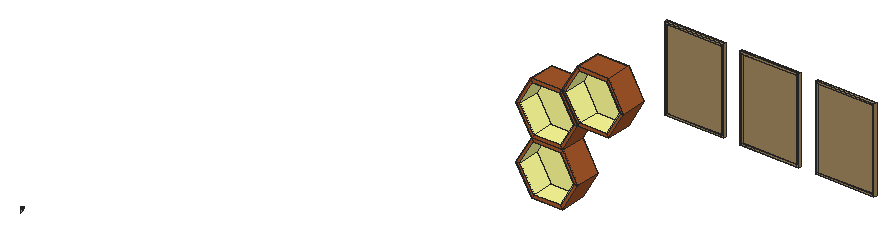
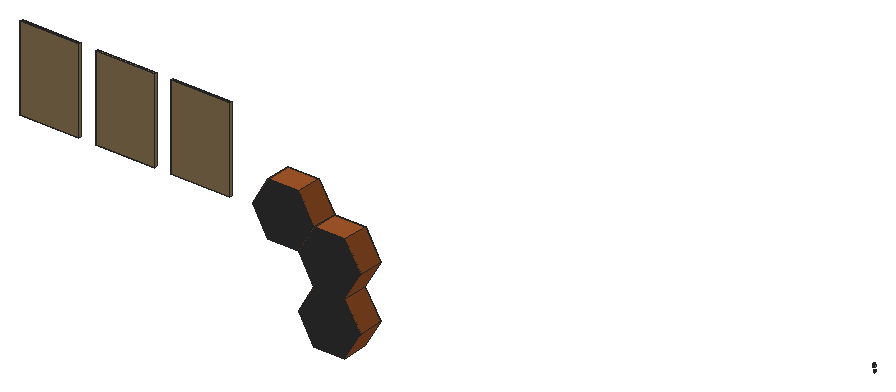
# SketchUp Ruby script. Lengths in inches.
U = 1.inch
M = Sketchup.active_model
def pt(a) = Geom::Point3d.new(a.map { |v| v * U })
def face(e, loops, mat)
  f = e.add_face(loops[0].map { |a| pt(a) })
  loops[1..].each { |l| e.add_face(l.map { |a| pt(a) }).erase! }
  f.material = f.back_material = mat if mat
  f
end
# faces: each face lists its corners as indices into pts; further lists are holes
def faces(e, pts, list, mat = nil) = list.each { |f| face(e, (f[0].is_a?(Array) ? f : [f]).map { |l| l.map { |i| pts[i] } }, mat) }
# xy, xz, yz: faces in a plane at the given z, y or x. An outline is a flat list of corners, or four numbers for a rectangle; further outlines are holes
def ring(l) = l.size == 4 ? [[l[0], l[1]], [l[2], l[1]], [l[2], l[3]], [l[0], l[3]]] : l.each_slice(2).to_a
def flat(e, list, mat, &to3) = list.each { |f| face(e, (f[0].is_a?(Array) ? f : [f]).map { |l| ring(l).map { |u, v| to3.(u, v) } }, mat) }
def xy(e, z, list, mat = nil) = flat(e, list, mat) { |x, y| [x, y, z] }
def xz(e, y, list, mat = nil) = flat(e, list, mat) { |x, z| [x, y, z] }
def yz(e, x, list, mat = nil) = flat(e, list, mat) { |y, z| [x, y, z] }
def lines(e, pts, list) = list.each { |a, b| e.add_line(pt(pts[a]), pt(pts[b])) }
# prism: a flat outline (further loops are holes) pulled along v
def prism(e, loops, v, mat = nil)
  f = face(e, loops, mat); d = Geom::Vector3d.new(v.map { |x| x * U })
  f.pushpull(f.normal.samedirection?(d) ? d.length : -d.length)
end
def box(e, o, s, mat = nil) = prism(e, [[o, [o[0] + s[0], o[1], o[2]], [o[0] + s[0], o[1] + s[1], o[2]], [o[0], o[1] + s[1], o[2]]]], [0, 0, s[2]], mat)
def at(x, y, z, deg = 0) = Geom::Transformation.translation(pt([x, y, z])) * Geom::Transformation.rotation(ORIGIN, Z_AXIS, deg.degrees)
def axes(o, x, y, z) = Geom::Transformation.new([*x, 0, *y, 0, *z, 0, *pt(o).to_a, 1])
def part(name) = M.definitions.add(name)
# library, detail: a bought-in or finely detailed component or shape, given as its bounding box
def library(name, o, s) = part(name).tap { |d| box(d.entities, o, s) }
def detail(e, o, s) = box(e.add_group.entities, o, s)
def put(e, d, t, mat = nil) = e.add_instance(d, t).tap { |i| i.material = mat if mat }
def group(e, t, mat = nil) = e.add_group.tap { |g| g.transformation = t; g.material = mat if mat }.entities
root = M.entities
M.materials.add("509740_G").color = [165, 87, 41]
M.materials.add("Laura_Hair").color = [160, 135, 94]
M.materials.add("[Color_007]").color = [58, 58, 58]
M.materials.add("[Color_E04]").color = [255, 255, 153]
M.materials.add("green").color = [174, 139, 102]
M.materials.add("vio").color = [206, 114, 100]
c1 = library("3DGeom~100_Defintion",[-500,-440.78,-130.77],[1000,881.57,261.54])
c2 = part("3DGeom~101_Defintion")
p = [[450.26,-438.5,-76.98],[473.93,-418.23,-130.77],[473.01,-420.54,-57.59],[450.72,-437.34,-113.57],[473.93,-418.23,-130.77],[450.26,-438.5,-76.98],
  [473.93,-418.23,-130.77],[450.72,-437.34,-113.57],[460.6,-429.08,-126.5],[473.01,-420.54,-57.59],[473.93,-418.23,-130.77],[496.21,-401.44,-74.78],
  [473.93,-418.23,-130.77],[487.14,-407.6875,-125.23],[496.68,-400.28,-111.37],[473.93,-418.23,-130.77],[496.68,-400.28,-111.37],[450.72,-437.34,-113.57],
  [450.26,-438.5,-76.98],[446.9375,-440.78,-95.45],[496.68,-400.28,-111.37],[500,-397.99,-92.9],[450.26,-438.5,-76.98],[473.01,-420.54,-57.59],
  [459.8,-431.09,-63.125],[473.01,-420.54,-57.59],[486.33,-409.69,-61.85],[-483.04,428.3125,67.76],[-497.53,394.8,97.99],[-487.96,391.61,113.91],
  [-483.04,428.3125,67.76],[-487.96,391.61,113.91],[-473.84,395.01,125.91],[-483.04,428.3125,67.76],[-500,403.73,82.41],[-497.53,394.8,97.99],
  [-483.04,428.3125,67.76],[-473.84,395.01,125.91],[-458.96,404.09,130.77],[-483.04,428.3125,67.76],[-494.7,415.99,71.34],[-483.04,428.3125,67.76],
  [-458.96,404.09,130.77],[-447.31,416.41,127.18],[-483.04,428.3125,67.76],[-447.31,416.41,127.18],[-442,428.67,116.12],[-483.04,428.3125,67.76],
  [-444.47,437.6,100.54],[-454.05,440.79,84.62],[-483.04,428.3125,67.76],[-454.05,440.79,84.62],[-468.16,437.39,72.62],[-483.04,428.3125,67.76],
  [-442,428.67,116.12],[-444.47,437.6,100.54]]
faces(c2.entities,p,[[0,1,2],[3,4,5],[6,7,8],[9,10,11],[12,13,14],[11,15,16],[17,18,19],[11,20,21],
  [22,23,24],[25,11,26],[27,28,29],[30,31,32],[33,34,35],[36,37,38],[39,40,34],[41,42,43],
  [44,45,46],[47,48,49],[50,51,52],[53,54,55]],"green")
c3 = part("3DGeom~221_Defintion")
p = [[192.89,-154.12,-424.75],[-160.54,-146.25,-441.73],[24.02,0,-500],[348.39,12.78,-359.13],[-312.36,-12.78,-390.87],[-151.29,154.12,-441.28],
  [202.15,146.25,-424.3],[348.39,12.78,-359.13],[-14.3,-279.72,-376.55],[-302.09,-253.31,-265.09],[-389.74,-176.26,-235.73],[-389.74,-176.26,-235.73],
  [-429.08,84.92,-237.62],[-429.08,84.92,-237.62],[-286.06,266.94,-264.32],[50.33,279.72,-373.45],[50.33,279.72,-373.45],[-286.06,266.94,-264.32],
  [310.08,-266.94,-235.68],[449.88,-84.92,-195.39],[310.08,-266.94,-235.68],[192.89,-154.12,-424.75],[192.89,-154.12,-424.75],[348.39,12.78,-359.13],
  [410.54,176.26,-197.28],[202.15,146.25,-424.3],[326.11,253.31,-234.91],[50.33,279.72,-373.45],[202.15,146.25,-424.3],[326.11,253.31,-234.91],
  [-312.36,-12.78,-390.87],[-389.74,-176.26,-235.73],[-457.125,-119.85,-147.25],[-312.36,-12.78,-390.87],[-429.08,84.92,-237.62],[87.19,-377.43,-212.82],
  [-217.65,-330.375,-227.46],[-14.3,-279.72,-376.55],[310.08,-266.94,-235.68],[87.19,-377.43,-212.82],[-217.65,-330.375,-227.46],[326.11,253.31,-234.91],
  [50.33,279.72,-373.45],[238.45,330.375,-205.55],[50.33,279.72,-373.45],[-286.06,266.94,-264.32],[-66.39,377.43,-220.19],[238.45,330.375,-205.55],
  [50.33,279.72,-373.45],[-66.39,377.43,-220.19],[469.14,119.85,-102.75],[-302.09,-253.31,-265.09],[-217.65,-330.375,-227.46],[-362.6875,-292.5,-17.42],
  [-302.09,-253.31,-265.09],[-362.6875,-292.5,-17.42],[-286.06,266.94,-264.32],[-479.41,120.6875,-23.03],[-286.06,266.94,-264.32],[-344.18,308.23,-16.53],
  [-286.06,266.94,-264.32],[-344.18,308.23,-16.53],[-486.1875,-99.2,-23.36],[344.18,-308.23,16.53],[87.19,-377.43,-212.82],[310.08,-266.94,-235.68],
  [479.41,-120.6875,23.03],[344.18,-308.23,16.53],[-362.6875,-292.5,-17.42],[362.6875,292.5,17.42],[238.45,330.375,-205.55],[-217.65,-330.375,-227.46],
  [-159.06,-386.79,-132.93],[-362.6875,-292.5,-17.42],[87.19,-377.43,-212.82],[-217.65,-330.375,-227.46],[-116.72,413.19,-5.61],[171.07,386.79,-117.07],
  [116.72,-413.19,5.61],[87.19,-377.43,-212.82],[344.18,-308.23,16.53],[87.19,-377.43,-212.82],[362.6875,292.5,17.42],[486.1875,99.2,23.36],
  [-362.6875,-292.5,-17.42],[-142.01,-407.43,-6.82],[142.01,407.43,6.82],[362.6875,292.5,17.42],[-469.14,-119.85,102.75],[-362.6875,-292.5,-17.42],
  [-449.88,84.92,195.39],[-344.18,308.23,-16.53],[-171.07,-386.79,117.07],[-238.45,-330.375,205.55],[-238.45,-330.375,205.55],[-326.11,-253.31,234.91],
  [-362.6875,-292.5,-17.42],[-410.54,-176.26,197.28],[-362.6875,-292.5,-17.42],[-326.11,-253.31,234.91],[-362.6875,-292.5,-17.42],[-344.18,308.23,-16.53],
  [-310.08,266.94,235.68],[-310.08,266.94,235.68],[66.39,-377.43,220.2],[-310.08,266.94,235.68],[-87.19,377.43,212.82],[286.06,-266.94,264.32],
  [286.06,-266.94,264.32],[344.18,-308.23,16.53],[159.06,386.79,132.93],[362.6875,292.5,17.42],[429.08,-84.92,237.62],[286.06,-266.94,264.32],
  [457.125,119.85,147.25],[389.74,176.26,235.73],[302.09,253.31,265.09],[217.65,330.375,227.46],[217.65,330.375,227.46],[362.6875,292.5,17.42],
  [-50.33,-279.72,373.45],[-50.33,-279.72,373.45],[14.3,279.72,376.55],[14.3,279.72,376.55],[217.65,330.375,227.46],[-348.39,-12.78,359.13],
  [-310.08,266.94,235.68],[-348.39,-12.78,359.13],[-348.39,-12.78,359.13],[-326.11,-253.31,234.91],[-202.15,-146.25,424.3],[-326.11,-253.31,234.91],
  [-238.45,-330.375,205.55],[-238.45,-330.375,205.55],[-50.33,-279.72,373.45],[-87.19,377.43,212.82],[-310.08,266.94,235.68],[-192.89,154.12,424.75],
  [-87.19,377.43,212.82],[14.3,279.72,376.55],[151.29,-154.12,441.28],[66.39,-377.43,220.2],[66.39,-377.43,220.2],[286.06,-266.94,264.32],
  [217.65,330.375,227.46],[160.54,146.25,441.73],[217.65,330.375,227.46],[302.09,253.31,265.09],[-348.39,-12.78,359.13],[-326.11,-253.31,234.91],
  [-202.15,-146.25,424.3],[312.36,12.78,390.87],[-310.08,266.94,235.68],[-348.39,-12.78,359.13],[-192.89,154.12,424.75],[302.09,253.31,265.09],
  [312.36,12.78,390.87],[389.74,176.26,235.73],[312.36,12.78,390.87],[286.06,-266.94,264.32],[429.08,-84.92,237.62],[312.36,12.78,390.87],
  [286.06,-266.94,264.32],[302.09,253.31,265.09],[312.36,12.78,390.87],[-348.39,-12.78,359.13],[-24.02,0,500],[312.36,12.78,390.87]]
faces(c3.entities,p,[[0,1,2],[3,0,2],[2,1,4],[2,4,5],[6,2,5],[7,2,6],[8,9,1],[0,8,1],
  [1,9,10],[1,11,4],[5,4,12],[5,13,14],[6,5,15],[16,5,17],[18,8,0],[19,20,21],
  [19,22,23],[24,23,25],[26,6,27],[24,28,29],[30,31,32],[33,32,34],[35,36,37],[38,39,8],
  [8,40,9],[41,42,43],[44,45,46],[47,48,49],[50,19,23],[50,23,24],[51,52,53],[31,54,55],
  [56,34,57],[58,57,59],[49,60,61],[34,32,62],[34,62,57],[63,64,65],[66,67,20],[32,31,68],
  [66,20,19],[24,29,69],[29,70,69],[71,72,73],[74,72,75],[49,61,76],[47,49,77],[77,49,76],
  [78,72,79],[80,78,81],[47,77,82],[50,24,69],[83,66,19],[83,19,50],[62,32,84],[78,85,72],
  [72,85,73],[77,86,87],[77,76,86],[83,50,69],[88,62,89],[57,62,88],[57,88,90],[91,57,90],
  [85,92,73],[92,93,73],[94,95,96],[97,88,98],[99,97,100],[101,90,102],[76,61,103],[104,85,78],
  [104,92,85],[76,105,106],[86,76,106],[107,104,78],[108,78,109],[86,110,111],[86,106,110],[112,113,67],
  [112,67,66],[114,83,69],[115,114,69],[116,115,69],[117,116,69],[110,118,119],[114,112,66],[114,66,83],
  [90,88,97],[120,93,92],[121,92,104],[110,106,122],[110,123,124],[115,112,114],[90,97,125],[126,90,127],
  [128,97,129],[130,131,132],[130,133,134],[135,136,137],[138,137,139],[140,134,141],[140,142,143],[144,139,145],
  [146,145,147],[148,149,150],[115,151,112],[152,153,154],[155,156,157],[158,159,160],[161,140,162],[163,145,164],
  [137,165,130],[166,130,134],[166,134,140],[139,137,166],[139,166,145],[145,140,167],[137,130,166],[145,166,140]],"vio")
c4 = library("3DGeom~121_Defintion",[-425.32,-500,-417.04],[850.64,1000,834.08])
c5 = part("3DGeom~122_Defintion")
p = [[-352.95,-477.04,-406.33],[-422.05,-474.42,-360.32],[-383.91,-455.37,-417.04],[-352.95,-477.04,-406.33],[-383.91,-455.37,-417.04],[-365.48,-464.73,-416.07],
  [-383.91,-455.37,-417.04],[-422.05,-474.42,-360.32],[-418.46,-454.05,-394.04],[-383.91,-455.37,-417.04],[-418.46,-454.05,-394.04],[-403.3,-451.46,-408.98],
  [-356.54,-497.41,-372.61],[-422.05,-474.42,-360.32],[-352.95,-477.04,-406.33],[-356.54,-497.41,-372.61],[-352.95,-477.04,-406.33],[-349.67,-489,-390.42],
  [-422.05,-474.42,-360.32],[-425.32,-462.46,-376.23],[-418.46,-454.05,-394.04],[-391.09,-496.09,-349.6],[-356.54,-497.41,-372.61],[-371.7,-500,-357.67],
  [-391.09,-496.09,-349.6],[-422.05,-474.42,-360.32],[-356.54,-497.41,-372.61],[-422.05,-474.42,-360.32],[-391.09,-496.09,-349.6],[-409.52,-486.73,-350.57],
  [376.78,485.85,408.43],[420.34,458.37,345.52],[409.52,472.35,336.91],[376.78,485.85,408.43],[409.52,472.35,336.91],[395.77,486.26,339.03],
  [376.78,485.85,408.43],[395.77,486.26,339.03],[382.76,496.38,351.32],[376.78,485.85,408.43],[425.32,448.07,362.5625],[420.34,458.37,345.52],
  [376.78,485.85,408.43],[382.76,496.38,351.32],[373.99,500,370.48],[376.78,485.85,408.43],[423.13,444.22,383.47],[376.78,485.85,408.43],
  [373.99,500,370.48],[371.8,496.14,391.39],[376.78,485.85,408.43],[414.36,447.84,402.63],[423.13,444.22,383.47],[376.78,485.85,408.43],
  [401.35,457.96,414.92],[414.36,447.84,402.63],[376.78,485.85,408.43],[387.6,471.87,417.04],[401.35,457.96,414.92]]
faces(c5.entities,p,[[0,1,2],[3,4,5],[6,7,8],[9,10,11],[12,13,14],[15,16,17],[18,19,20],[21,22,23],
  [24,25,26],[27,28,29],[30,31,32],[33,34,35],[36,37,38],[39,40,41],[42,43,44],[45,46,40],
  [47,48,49],[50,51,52],[53,54,55],[56,57,58]],"green")
c6 = part("3DGeom~227_Defintion")
p = [[-46.82,-86.11,-495.11],[-183.22,-312.53,-297.48],[-255.21,-122.37,-414.37],[57.41,-270.66,-390.71],[148.25,12.96,-485.1875],[-138.51,121.52,-466.84],
  [-25.88,178.72,-461.11],[282.66,-156.27,-379.26],[277.73,148.29,-387.25],[48.875,256.85,-404.57],[-258.82,100.58,-420.23],[-193.08,296.58,-313.48],
  [-421.09,-86.11,-264.6],[-421.09,-86.11,-264.6],[-354.59,121.52,-333.75],[-255.21,-122.37,-414.37],[-183.22,-312.53,-297.48],[-374.76,-270.66,-124.54],
  [-255.21,-122.37,-414.37],[-421.09,-86.11,-264.6],[65.73,334.98,-312.37],[57.41,-270.66,-390.71],[-62.14,-418.95,-100.89],[-183.22,-312.53,-297.48],
  [57.41,-270.66,-390.71],[146.25,-382.69,-181.63],[146.25,-382.69,-181.63],[432.17,0,-266.17],[306.92,283.62,-227.56],[432.17,0,-266.17],
  [277.73,148.29,-387.25],[306.92,283.62,-227.56],[341.32,-283.625,-171.7],[146.25,-382.69,-181.63],[432.17,0,-266.17],[341.32,-283.625,-171.7],
  [282.66,-156.27,-379.26],[-354.59,121.52,-333.75],[-500,12.96,-85.92],[-354.59,121.52,-333.75],[-400.15,178.72,-230.6],[-400.15,178.72,-230.6],
  [-383.29,256.85,-138.4],[-193.08,296.58,-313.48],[-383.29,256.85,-138.4],[-308.54,334.98,-81.86],[-193.08,296.58,-313.48],[-195.91,392.18,-76.125],
  [-193.08,296.58,-313.48],[-75.6,413.11,-122.74],[-193.08,296.58,-313.48],[20.17,392.18,-209.21],[65.73,334.98,-312.37],[-193.08,296.58,-313.48],
  [-193.08,296.58,-313.48],[306.92,283.62,-227.56],[65.73,334.98,-312.37],[-183.22,-312.53,-297.48],[-228.01,-382.69,48.88],[-183.22,-312.53,-297.48],
  [-228.01,-382.69,48.88],[-374.76,-270.66,-124.54],[432.17,0,-266.17],[470.8,-148.29,-73.77],[341.32,-283.625,-171.7],[465.88,156.27,-81.77],
  [432.17,0,-266.17],[306.92,283.62,-227.56],[432.17,0,-266.17],[-465.88,-156.27,81.77],[-470.8,148.29,73.77],[-383.29,256.85,-138.4],
  [228.01,382.69,-48.88],[306.92,283.62,-227.56],[228.01,382.69,-48.88],[306.92,283.62,-227.56],[75.6,-413.11,122.74],[195.91,-392.18,76.125],
  [341.32,-283.625,-171.7],[341.32,-283.625,-171.7],[308.54,-334.98,81.86],[308.54,-334.98,81.86],[341.32,-283.625,-171.7],[-383.29,256.85,-138.4],
  [-341.32,283.625,171.7],[-383.29,256.85,-138.4],[-341.32,283.625,171.7],[-308.54,334.98,-81.86],[-228.01,-382.69,48.88],[-306.92,-283.62,227.56],
  [62.14,418.95,100.89],[-20.17,-392.18,209.21],[-228.01,-382.69,48.88],[-432.17,0,266.17],[-341.32,283.625,171.7],[-146.25,382.69,181.63],
  [500,-12.96,85.92],[374.76,270.66,124.54],[228.01,382.69,-48.88],[383.29,-256.85,138.4],[308.54,-334.98,81.86],[374.76,270.66,124.54],
  [-228.01,-382.69,48.88],[-65.73,-334.98,312.37],[-228.01,-382.69,48.88],[-65.73,-334.98,312.37],[-306.92,-283.62,227.56],[-282.66,156.27,379.26],
  [-282.66,156.27,379.26],[-341.32,283.625,171.7],[193.08,-296.58,313.48],[-277.73,-148.29,387.25],[-277.73,-148.29,387.25],[383.29,-256.85,138.4],
  [400.15,-178.72,230.6],[421.09,86.11,264.6],[183.22,312.53,297.48],[374.76,270.66,124.54],[183.22,312.53,297.48],[193.08,-296.58,313.48],
  [-341.32,283.625,171.7],[-282.66,156.27,379.26],[-57.41,270.66,390.71],[-341.32,283.625,171.7],[-57.41,270.66,390.71],[-146.25,382.69,181.63],
  [-57.41,270.66,390.71],[-65.73,-334.98,312.37],[-306.92,-283.62,227.56],[-65.73,-334.98,312.37],[-48.875,-256.85,404.57],[-306.92,-283.62,227.56],
  [-277.73,-148.29,387.25],[400.15,-178.72,230.6],[354.59,-121.52,333.75],[193.08,-296.58,313.48],[354.59,-121.52,333.75],[255.21,122.37,414.37],
  [354.59,-121.52,333.75],[421.09,86.11,264.6],[183.22,312.53,297.48],[255.21,122.37,414.37],[-432.17,0,266.17],[-148.25,-12.96,485.1875],
  [-432.17,0,266.17],[-57.41,270.66,390.71],[255.21,122.37,414.37],[183.22,312.53,297.48],[193.08,-296.58,313.48],[25.88,-178.72,461.11],
  [193.08,-296.58,313.48],[138.51,-121.52,466.84],[193.08,-296.58,313.48],[258.82,-100.58,420.23],[193.08,-296.58,313.48],[354.59,-121.52,333.75],
  [193.08,-296.58,313.48],[255.21,122.37,414.37],[354.59,-121.52,333.75],[46.82,86.11,495.11],[-57.41,270.66,390.71],[-57.41,270.66,390.71],
  [255.21,122.37,414.37],[255.21,122.37,414.37]]
faces(c6.entities,p,[[0,1,2],[0,3,1],[4,3,0],[5,0,2],[6,0,5],[6,4,0],[4,7,3],[8,7,4],
  [9,4,6],[9,8,4],[5,2,10],[5,10,11],[6,5,11],[9,6,11],[10,2,12],[10,13,14],
  [10,14,11],[15,16,17],[18,17,19],[20,8,9],[20,9,11],[21,22,23],[24,25,22],[7,26,3],
  [8,27,7],[28,29,30],[20,31,8],[7,32,33],[34,35,36],[37,19,38],[39,38,40],[14,41,11],
  [40,42,43],[44,45,46],[45,47,48],[47,49,50],[51,52,53],[49,51,54],[51,55,56],[57,22,58],
  [59,60,61],[62,63,64],[65,63,66],[67,65,68],[19,17,69],[19,69,38],[40,38,70],[40,70,71],
  [72,65,73],[51,74,75],[49,74,51],[25,76,22],[25,77,76],[78,77,25],[79,80,77],[63,81,82],
  [83,70,84],[85,86,87],[17,88,89],[17,89,69],[49,90,74],[47,90,49],[22,91,92],[22,76,91],
  [38,69,93],[38,93,70],[45,94,95],[45,95,47],[65,96,63],[97,96,65],[98,97,65],[47,95,90],
  [63,99,100],[96,99,63],[90,101,74],[102,91,103],[104,105,106],[70,93,107],[70,108,109],[76,77,110],
  [77,80,110],[69,89,111],[69,112,93],[80,113,110],[96,114,99],[115,114,96],[97,115,96],[90,116,117],
  [95,116,90],[91,76,110],[118,115,97],[99,114,119],[120,121,122],[123,124,125],[95,126,116],[127,91,110],
  [128,129,130],[131,130,132],[133,134,135],[115,136,114],[137,138,139],[140,141,115],[142,132,143],[144,143,121],
  [145,146,147],[130,129,148],[149,130,150],[151,149,152],[153,151,154],[155,153,156],[157,153,158],[121,143,159],
  [121,159,160],[132,130,149],[132,149,143],[161,159,162],[159,153,163],[159,151,153],[143,149,151],[143,151,159]],"vio")
c7 = part("Group\#32")
xy(c7.entities,0,[[3.62,0,10.87,5.91]],"509740_G")
xy(c7.entities,0.79,[[4.08,0,10.41,5.12]],"[Color_E04]")
xy(c7.entities,11.8125,[[4.08,0,10.41,5.12]],"[Color_E04]")
xy(c7.entities,12.6,[[3.62,0,10.87,5.91]],"509740_G")
xz(c7.entities,0,[[3.62,0,4.08,0.79,0.91,6.3,0,6.3],[3.62,0,10.87,0,10.41,0.79,4.08,0.79],[10.87,0,14.49,6.3,13.58,6.3,10.41,0.79],[0,6.3,0.91,6.3,4.08,11.8125,3.62,12.6],[13.58,6.3,14.49,6.3,10.87,12.6,10.41,11.8125],
  [4.08,11.8125,10.41,11.8125,10.87,12.6,3.62,12.6]],"509740_G")
xz(c7.entities,5.12,[[4.08,0.79,10.41,0.79,13.58,6.3,10.41,11.8125,4.08,11.8125,0.91,6.3]],"[Color_E04]")
xz(c7.entities,5.91,[[3.62,0,0,6.3,3.62,12.6,10.87,12.6,14.49,6.3,10.87,0]],"[Color_007]")
p = [[0,5.91,6.3],[3.62,5.91,0],[3.62,0,0],[0,0,6.3],[10.87,5.91,0],[14.49,5.91,6.3],
  [14.49,0,6.3],[10.87,0,0],[0.91,0,6.3],[4.08,0,0.79],[4.08,5.12,0.79],[0.91,5.12,6.3],
  [10.41,0,0.79],[13.58,0,6.3],[13.58,5.12,6.3],[10.41,5.12,0.79],[3.62,5.91,12.6],[3.62,0,12.6],
  [4.08,0,11.8125],[4.08,5.12,11.8125],[10.41,0,11.8125],[10.41,5.12,11.8125],[10.87,5.91,12.6],[10.87,0,12.6]]
faces(c7.entities,p,[[0,1,2,3],[4,5,6,7],[16,0,3,17],[5,22,23,6]],"509740_G")
faces(c7.entities,p,[[8,9,10,11],[12,13,14,15],[18,8,11,19],[13,20,21,14]],"[Color_E04]")
c8 = part("WALL SHELVES 01")
g1 = group(c8.entities,at(13.71,-9.84,19.85))
put(g1,c7,at(0,0,0))
put(g1,c7,at(10.87,0,6.3))
put(g1,c7,at(21.73,0,0))
c9 = part("Plant Wall Art")
g2 = group(c9.entities,at(1.72,0.59,0))
xy(g2,0,[[0,-0.59,13.78,0]],"Laura_Hair")
xy(g2,0.39,[[0.39,-0.59,13.39,-0.39]],"Laura_Hair")
xy(g2,19.29,[[0.39,-0.59,13.39,-0.39]],"Laura_Hair")
xy(g2,19.69,[[0,-0.59,13.78,0]],"Laura_Hair")
xz(g2,-0.59,[[[0,0,13.78,19.69],[0.39,0.39,13.39,19.29]]],"Laura_Hair")
xz(g2,0,[[0,0,13.78,19.69]],"Laura_Hair")
yz(g2,0,[[-0.59,0,0,19.69]],"Laura_Hair")
yz(g2,0.39,[[-0.59,0.39,-0.39,19.29]],"Laura_Hair")
yz(g2,13.39,[[-0.59,0.39,-0.39,19.29]],"Laura_Hair")
yz(g2,13.78,[[-0.59,0,0,19.69]],"Laura_Hair")
p = [[13.39,0,0.39],[13.39,-0.39,0.39],[13.39,0,19.29],[13.39,-0.39,19.29],[0.39,0,0.39],[0.39,-0.39,0.39],
  [0.39,0,19.29],[0.39,-0.39,19.29]]
lines(g2,p,[[0,1],[2,3],[4,5],[6,7]])
g3 = group(c9.entities,at(19.43,0.59,0))
xy(g3,0,[[0,-0.59,13.78,0]],"Laura_Hair")
xy(g3,0.39,[[0.39,-0.59,13.39,-0.39]],"Laura_Hair")
xy(g3,19.29,[[0.39,-0.59,13.39,-0.39]],"Laura_Hair")
xy(g3,19.69,[[0,-0.59,13.78,0]],"Laura_Hair")
xz(g3,-0.59,[[[0,0,13.78,19.69],[0.39,0.39,13.39,19.29]]],"Laura_Hair")
xz(g3,0,[[0,0,13.78,19.69]],"Laura_Hair")
yz(g3,0,[[-0.59,0,0,19.69]],"Laura_Hair")
yz(g3,0.39,[[-0.59,0.39,-0.39,19.29]],"Laura_Hair")
yz(g3,13.39,[[-0.59,0.39,-0.39,19.29]],"Laura_Hair")
yz(g3,13.78,[[-0.59,0,0,19.69]],"Laura_Hair")
p = [[13.39,0,0.39],[13.39,-0.39,0.39],[13.39,0,19.29],[13.39,-0.39,19.29],[0.39,0,0.39],[0.39,-0.39,0.39],
  [0.39,0,19.29],[0.39,-0.39,19.29]]
lines(g3,p,[[0,1],[2,3],[4,5],[6,7]])
g4 = group(c9.entities,at(37.15,0.59,0))
xy(g4,0,[[0,-0.59,13.78,0]],"Laura_Hair")
xy(g4,0.39,[[0.39,-0.59,13.39,-0.39]],"Laura_Hair")
xy(g4,19.29,[[0.39,-0.59,13.39,-0.39]],"Laura_Hair")
xy(g4,19.69,[[0,-0.59,13.78,0]],"Laura_Hair")
xz(g4,-0.59,[[[0,0,13.78,19.69],[0.39,0.39,13.39,19.29]]],"Laura_Hair")
xz(g4,0,[[0,0,13.78,19.69]],"Laura_Hair")
yz(g4,0,[[-0.59,0,0,19.69]],"Laura_Hair")
yz(g4,0.39,[[-0.59,0.39,-0.39,19.29]],"Laura_Hair")
yz(g4,13.39,[[-0.59,0.39,-0.39,19.29]],"Laura_Hair")
yz(g4,13.78,[[-0.59,0,0,19.69]],"Laura_Hair")
p = [[13.39,0,0.39],[13.39,-0.39,0.39],[13.39,0,19.29],[13.39,-0.39,19.29],[0.39,0,0.39],[0.39,-0.39,0.39],
  [0.39,0,19.29],[0.39,-0.39,19.29]]
lines(g4,p,[[0,1],[2,3],[4,5],[6,7]])
g5 = group(root,at(15.3125,134.49,26.21))
put(g5,c1,axes([4.38,0.85,15.02],[0,0.0004,0],[0,0,-0.0004],[-0.0004,0,0]),"green")
put(g5,c2,axes([4.38,0.85,15.02],[0,0.0004,0],[0,0,-0.0004],[-0.0004,0,0]),"green")
g6 = group(root,at(15.3125,134.49,26.21))
put(g6,c3,axes([4.42,1.07,15.21],[0,0.00039,0],[0,0,-0.00039],[-0.00039,0,0]),"vio")
g7 = group(root,at(15.3125,134.49,26.21))
put(g7,c4,axes([4.85,0.57,15.95],[0,0.00036,0],[0,0,-0.00036],[-0.00036,0,0]),"green")
put(g7,c5,axes([4.85,0.57,15.95],[0,0.00036,0],[0,0,-0.00036],[-0.00036,0,0]),"green")
g8 = group(root,at(15.3125,134.49,26.21))
put(g8,c6,axes([5.01,0.41,16.15],[0,0.00038,0],[0,0,-0.00038],[-0.00038,0,0]),"vio")
put(root,c8,axes([141.71,201.9375,75.5],[-0.5,0,-0.86603],[0,1,0],[-0.86603,0,0.5]))
put(root,c9,at(119.41,197.41,69.8125))
